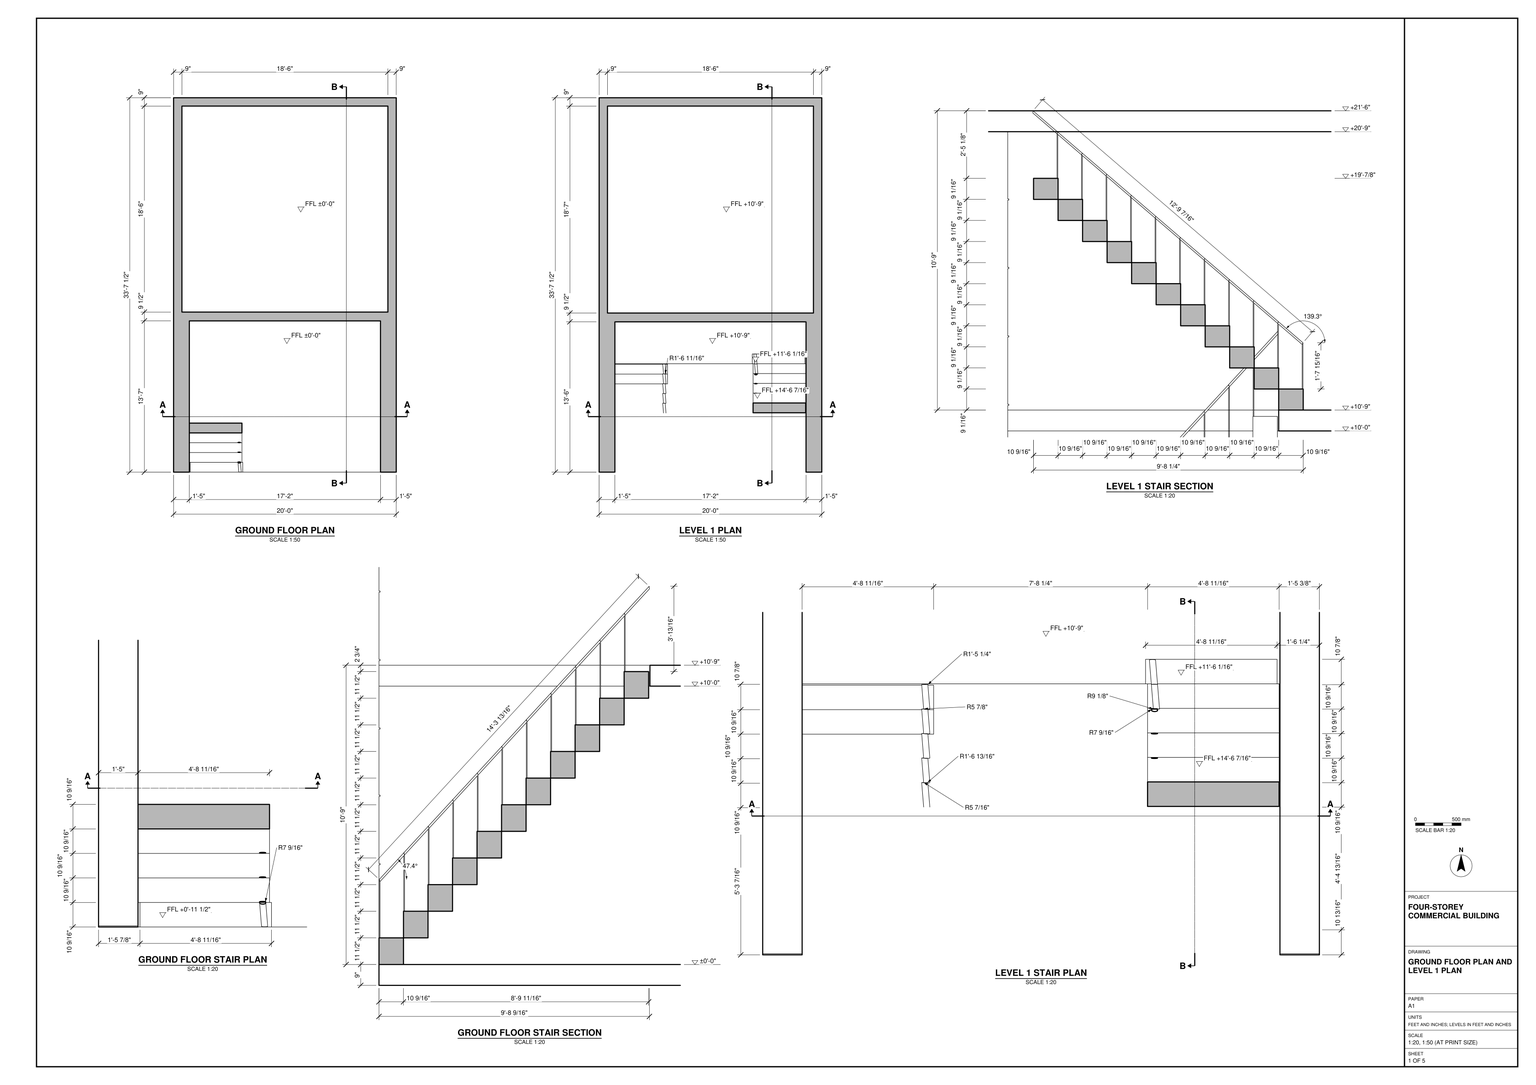
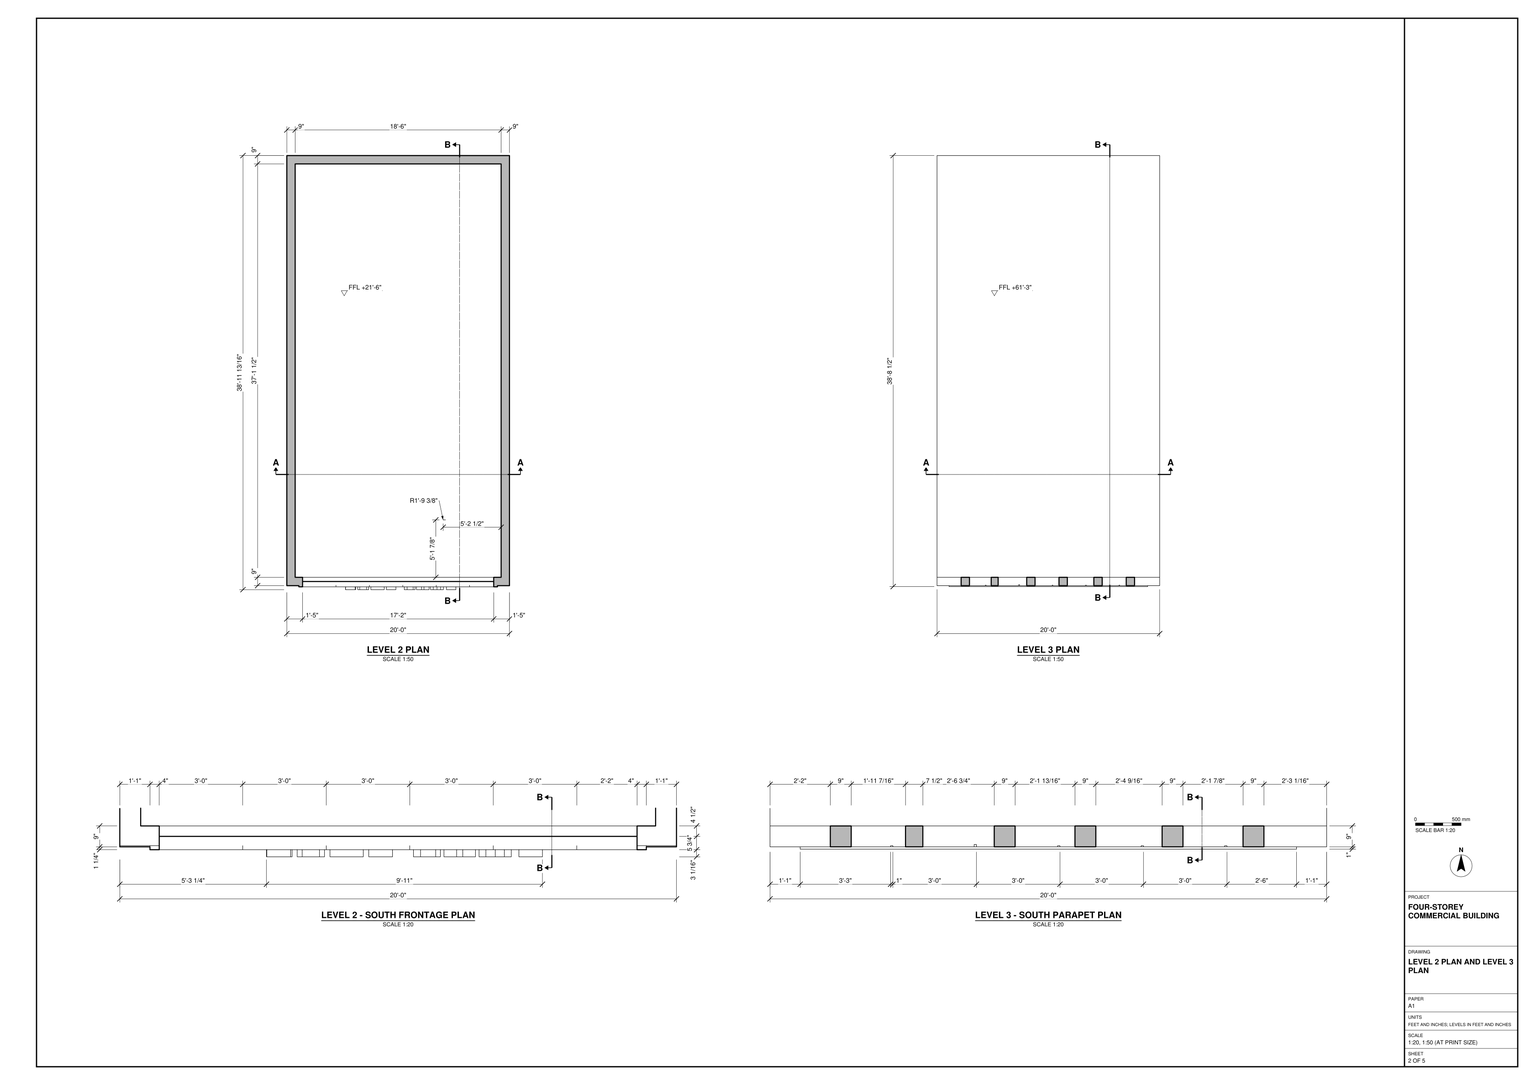
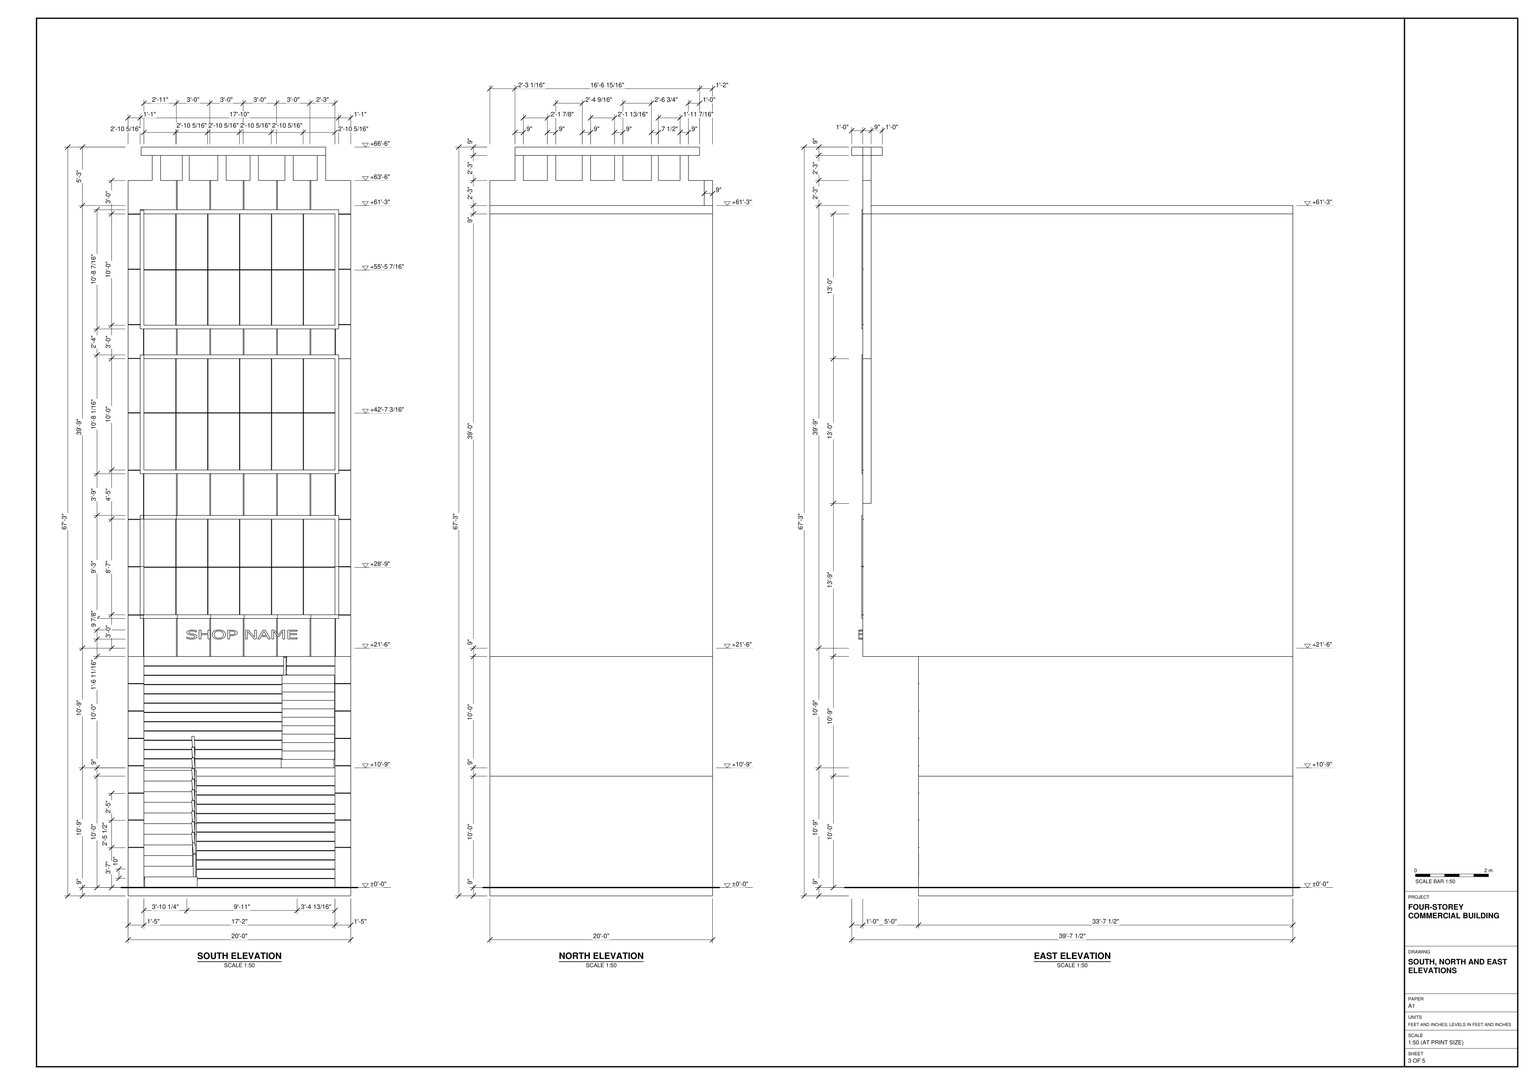
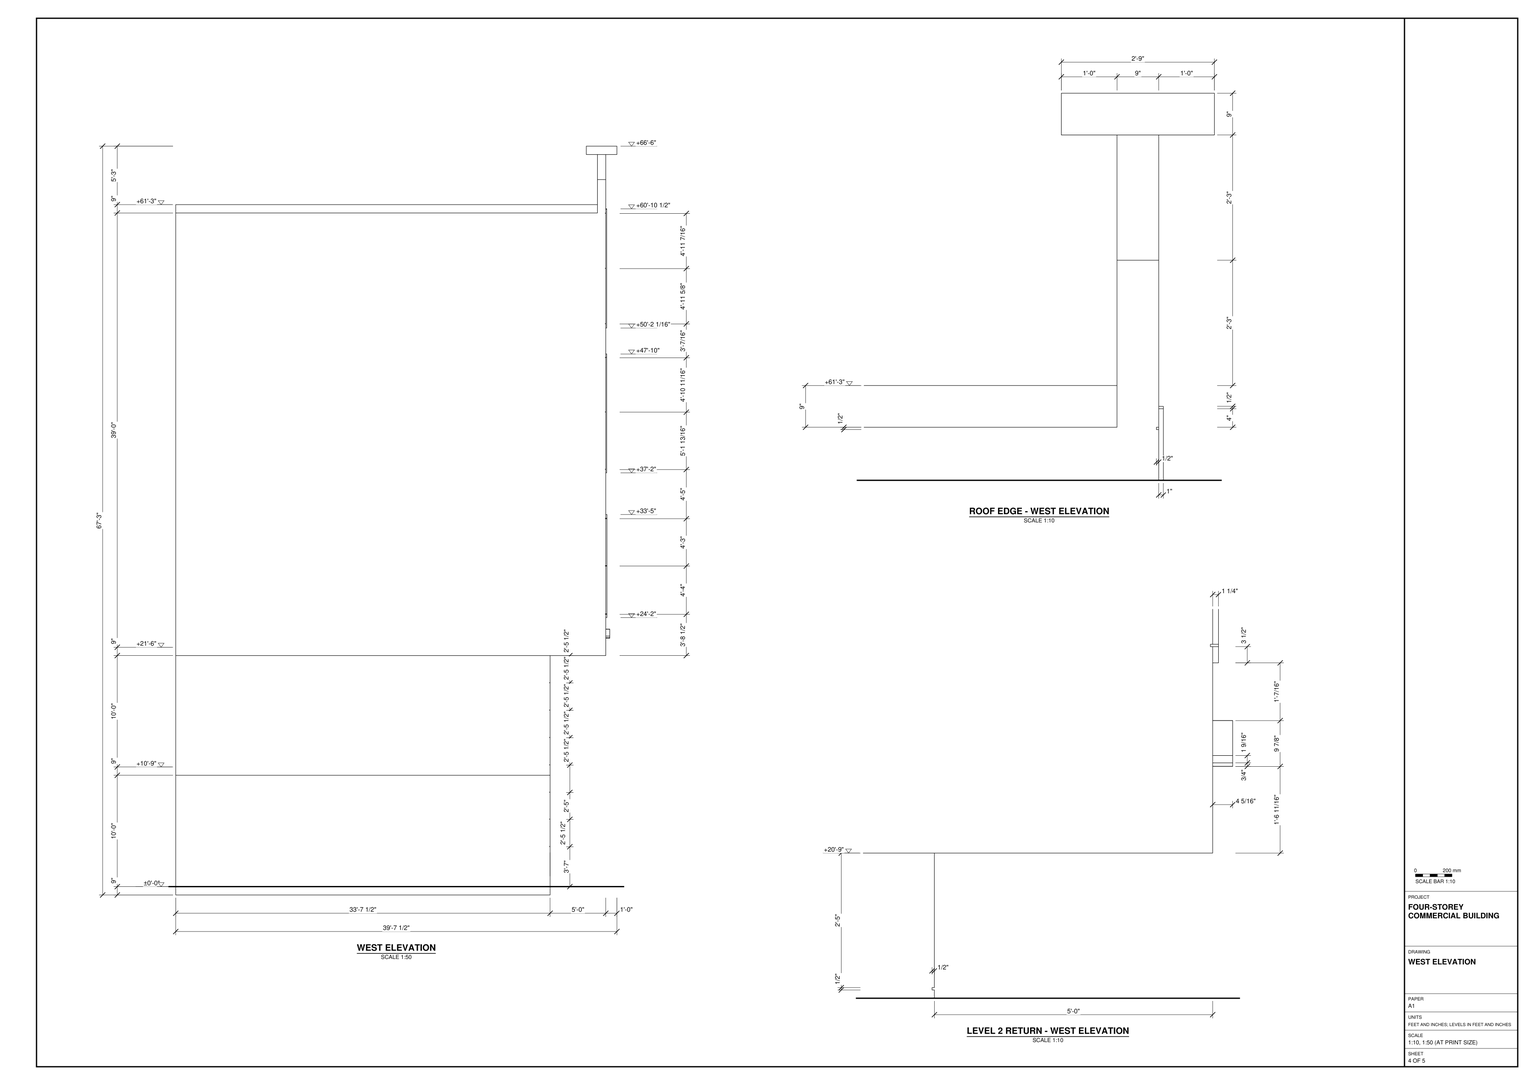
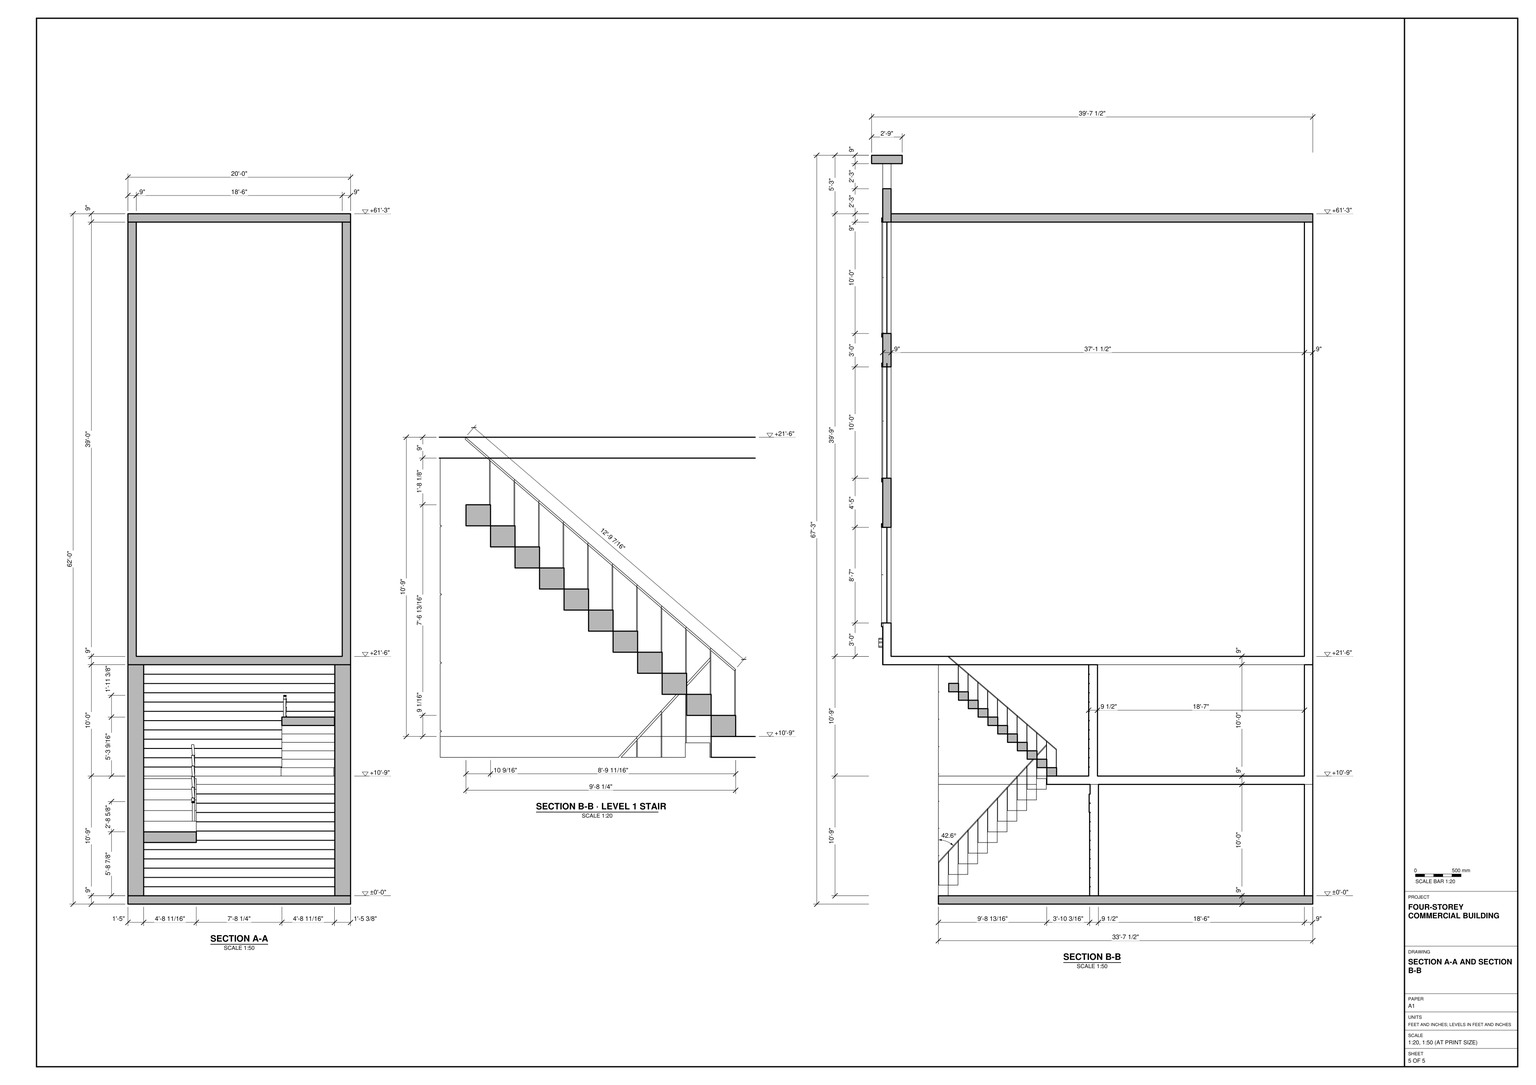
Build the commercial building in SketchUp from task_files/diagram_01.pdf. Work in feet and inches. The overall dimensions are 20'-0" across the south frontage, 39'-7 1/2" from front to back and 67'-3" from the underside of the base slab to the top of the parapet cap. Set the levels at ±0'-0", +10'-9", +21'-6" and +61'-3".

Use the ground and first-level plans to lay out the rear enclosure and the open stair bay to its south. Follow the wall thicknesses shown, including the 9" side walls around the rear space and the 1'-5" walls flanking the stair bay. Model the stair flights on the sides indicated in plan, with individual steps, landings, sloping handrails and upright supports. Use the east elevation to locate the lower setback and the upper volume that projects over it.

Model the floor slabs and flat roof. On the south face, place the shop sign in the band above the stair opening. Above it, build the three stacked glazed panels with their perimeter frames and internal divisions. Finish the south parapet with spaced uprights beneath a continuous cap. Group walls, slabs, roof and each furniture or joinery piece separately, and use components for repeated parts. Any decor or loose items shown may be suitable library components. Save one SketchUp model as output_files/four_storey_commercial_building_with_south_stair.skp.

# SketchUp Ruby script. Lengths in inches.
U = 1.inch
M = Sketchup.active_model
def pt(a) = Geom::Point3d.new(a.map { |v| v * U })
def face(e, loops, mat)
  f = e.add_face(loops[0].map { |a| pt(a) })
  loops[1..].each { |l| e.add_face(l.map { |a| pt(a) }).erase! }
  f.material = f.back_material = mat if mat
  f
end
# faces: each face lists its corners as indices into pts; further lists are holes
def faces(e, pts, list, mat = nil) = list.each { |f| face(e, (f[0].is_a?(Array) ? f : [f]).map { |l| l.map { |i| pts[i] } }, mat) }
# xy, xz, yz: faces in a plane at the given z, y or x. An outline is a flat list of corners, or four numbers for a rectangle; further outlines are holes
def ring(l) = l.size == 4 ? [[l[0], l[1]], [l[2], l[1]], [l[2], l[3]], [l[0], l[3]]] : l.each_slice(2).to_a
def flat(e, list, mat, &to3) = list.each { |f| face(e, (f[0].is_a?(Array) ? f : [f]).map { |l| ring(l).map { |u, v| to3.(u, v) } }, mat) }
def xy(e, z, list, mat = nil) = flat(e, list, mat) { |x, y| [x, y, z] }
def xz(e, y, list, mat = nil) = flat(e, list, mat) { |x, z| [x, y, z] }
def yz(e, x, list, mat = nil) = flat(e, list, mat) { |y, z| [x, y, z] }
def lines(e, pts, list) = list.each { |a, b| e.add_line(pt(pts[a]), pt(pts[b])) }
# prism: a flat outline (further loops are holes) pulled along v
def prism(e, loops, v, mat = nil)
  f = face(e, loops, mat); d = Geom::Vector3d.new(v.map { |x| x * U })
  f.pushpull(f.normal.samedirection?(d) ? d.length : -d.length)
end
def box(e, o, s, mat = nil) = prism(e, [[o, [o[0] + s[0], o[1], o[2]], [o[0] + s[0], o[1] + s[1], o[2]], [o[0], o[1] + s[1], o[2]]]], [0, 0, s[2]], mat)
def at(x, y, z, deg = 0) = Geom::Transformation.translation(pt([x, y, z])) * Geom::Transformation.rotation(ORIGIN, Z_AXIS, deg.degrees)
def axes(o, x, y, z) = Geom::Transformation.new([*x, 0, *y, 0, *z, 0, *pt(o).to_a, 1])
def part(name) = M.definitions.add(name)
# library, detail: a bought-in or finely detailed component or shape, given as its bounding box
def library(name, o, s) = part(name).tap { |d| box(d.entities, o, s) }
def detail(e, o, s) = box(e.add_group.entities, o, s)
def put(e, d, t, mat = nil) = e.add_instance(d, t).tap { |i| i.material = mat if mat }
def group(e, t, mat = nil) = e.add_group.tap { |g| g.transformation = t; g.material = mat if mat }.entities
root = M.entities
M.materials.add("Granite Dark Gray").color = [69, 68, 68]
M.materials.add("[0097_DeepSkyBlue]").color = [0, 191, 255]
M.materials.add("[0128_White]").color = [255, 255, 255]
M.materials.add("[0132_LightGray]").color = [169, 169, 169]
M.materials.add("[0134_DimGray]").color = [105, 105, 105]
M.materials.add("[0136_Charcoal]").color = [35, 35, 35]
M.materials.add("[0137_Black]").color = [0, 0, 0]
M.materials.add("[Formica Beige]").color = [211, 187, 149]
c1 = library("SHOP NAME",[0.49,0,0],[69.73,9.9,1])
c2 = part("Stair railing section")
xy(c2.entities,0,[[0,0,70.0625,99.4375]],"[0128_White]")
xy(c2.entities,31.125,[[0,0,70.0625,99.4375]],"[0132_LightGray]")
xz(c2.entities,0,[[0,0,70.0625,31.125]],"[0128_White]")
xz(c2.entities,99.4375,[[0,0,70.0625,31.125]],"[0128_White]")
yz(c2.entities,0,[[0,0,99.4375,31.125]],"[0128_White]")
yz(c2.entities,70.0625,[[0,0,99.4375,31.125]],"[0128_White]")
p = [[65.96,1.08,31.125],[66.39,1.03,31.125],[66.39,1.03,99.4],[65.96,1.08,99.35],[66.8125,1.08,31.125],[66.8125,1.08,99.36],
  [65.56,1.25,31.125],[65.56,1.25,99.23],[67.21,1.25,31.125],[67.21,1.25,99.24],[65.22,1.51,31.125],[65.22,1.51,99.03],
  [67.55,1.51,31.125],[67.55,1.51,99.05],[64.96,1.85,31.125],[64.96,1.85,98.78],[67.8125,1.85,31.125],[67.8125,1.85,98.8],
  [64.8,2.24,31.125],[64.8,2.24,98.49],[67.98,2.24,31.125],[67.98,2.24,98.51],[64.74,2.67,31.125],[64.74,2.67,98.17],
  [68.03,2.67,31.125],[68.03,2.67,98.2],[64.8,3.1,31.125],[64.8,3.1,97.86],[67.98,3.1,31.125],[67.98,3.1,97.89],
  [64.96,3.49,31.125],[64.96,3.49,97.57],[67.8125,3.49,31.125],[67.8125,3.49,97.59],[65.22,3.83,31.125],[65.22,3.83,97.32],
  [67.55,3.83,31.125],[67.55,3.83,97.34],[65.56,4.09,31.125],[65.56,4.09,97.13],[67.21,4.09,31.125],[67.21,4.09,97.15],
  [65.96,4.26,31.125],[65.96,4.26,97.02],[66.8125,4.26,31.125],[66.8125,4.26,97.02],[66.39,4.31,31.125],[66.39,4.31,96.98],
  [64.51,102.53,127.95],[64.91,102.58,127.79],[65.76,102.59,127.8],[66.16,102.54,127.96],[65.34,102.6,127.74],[64.17,102.45,128.19],
  [66.5,102.46,128.21],[63.91,102.34,128.51],[66.75,102.36,128.54],[63.74,102.22,128.89],[66.92,102.25,128.92],[63.68,102.1,129.3],
  [66.97,102.12,129.33],[63.73,101.97,129.7],[66.91,101.99,129.73],[63.89,101.85,130.08],[66.74,101.87,130.11],[64.15,101.75,130.41],
  [66.48,101.77,130.43],[64.49,101.68,130.66],[66.14,101.6875,130.68],[64.89,101.63,130.82],[65.74,101.64,130.83],[65.3125,101.62,130.88]]
faces(c2.entities,p,[[0,1,2,3],[1,4,5,2],[6,0,3,7],[4,8,9,5],[10,6,7,11],[8,12,13,9],[14,10,11,15],[12,16,17,13],
  [18,14,15,19],[16,20,21,17],[22,18,19,23],[20,24,25,21],[26,22,23,27],[24,28,29,25],[30,26,27,31],[28,32,33,29],
  [34,30,31,35],[32,36,37,33],[38,34,35,39],[36,40,41,37],[42,38,39,43],[40,44,45,41],[46,42,43,47],[44,46,47,45],
  [43,39,48,49],[41,45,50,51],[47,43,49,52],[45,47,52,50],[39,35,53,48],[37,41,51,54],[35,31,55,53],[33,37,54,56],
  [31,27,57,55],[29,33,56,58],[27,23,59,57],[25,29,58,60],[23,19,61,59],[21,25,60,62],[19,15,63,61],[17,21,62,64],
  [15,11,65,63],[13,17,64,66],[11,7,67,65],[9,13,66,68],[7,3,69,67],[5,9,68,70],[3,2,71,69],[2,5,70,71]],"[0128_White]")
c3 = part("Group\#4")
xz(c3.entities,0,[[0,0,34.33,51],[34.83,0,68.67,51],[69.17,0,103,51],[103.5,0,137.33,51],[137.83,0,171.67,51],
  [172.17,0,206,51],[0,51.5,34.33,103],[34.83,51.5,68.67,103],[69.17,51.5,103,103],[103.5,51.5,137.33,103],
  [137.83,51.5,171.67,103],[172.17,51.5,206,103]],"[0097_DeepSkyBlue]")
xz(c3.entities,0,[[34.33,0,34.83,51],[68.67,0,69.17,51],[103,0,103.5,51],[137.33,0,137.83,51],[171.67,0,172.17,51],
  [0,51,34.33,51.5],[34.33,51,34.83,51.5],[34.83,51,68.67,51.5],[68.67,51,69.17,51.5],[69.17,51,103,51.5],
  [103,51,103.5,51.5],[103.5,51,137.33,51.5],[137.33,51,137.83,51.5],[137.83,51,171.67,51.5],[171.67,51,172.17,51.5],
  [172.17,51,206,51.5],[34.33,51.5,34.83,103],[68.67,51.5,69.17,103],[103,51.5,103.5,103],[137.33,51.5,137.83,103],
  [171.67,51.5,172.17,103]],"[0137_Black]")
xy(root,-9,[[0,72,240,475.51]])
xy(root,0,[[[0,72,0,475.51,240,475.51,240,72,223,72,223,235.01,17,235.01,17,72],[9,244.51,231,466.51]],[17,72,223,235.01],[9,244.51,231,466.51]])
xy(root,9.5,[[17,235,223,235.5]])
xy(root,10,[[17,235,223,235.5]])
xy(root,19.5,[[17,235,223,235.5]])
xy(root,20,[[17,235,223,235.5]])
xy(root,29.5,[[17,235,223,235.5]])
xy(root,30,[[17,235,223,235.5]])
xy(root,39.5,[[17,235,223,235.5]])
xy(root,40,[[17,235,223,235.5]])
xy(root,43,[[0,72,17,72.5],[223,72,240,72.5]],"[Formica Beige]")
xy(root,43.5,[[0,72,17,72.5],[223,72,240,72.5]],"[Formica Beige]")
xy(root,49.5,[[17,234.99,223,235.5]])
xy(root,50,[[17,234.99,223,235.5]])
xy(root,59.5,[[17,234.99,223,235.49]])
xy(root,60,[[17,234.99,223,235.49]])
xy(root,69.5,[[17,234.99,223,235.49]])
xy(root,70,[[17,234.99,223,235.49]])
xy(root,72.5,[[0,72,17,72.5],[223,72,240,72.5]],"[Formica Beige]")
xy(root,73,[[0,72,17,72.5],[223,72,240,72.5]],"[Formica Beige]")
xy(root,79.5,[[17,234.99,223,235.49]])
xy(root,80,[[17,234.99,223,235.49]])
xy(root,89.5,[[17,234.99,223,235.49]])
xy(root,90,[[17,234.49,223,235.49]])
xy(root,99.5,[[17,234.48,223,235.48]])
xy(root,100,[[17,234.48,223,235.48]])
xy(root,101.5,[[0,72,17,72.5],[223,72,240,72.5]],"[Formica Beige]")
xy(root,102,[[0,72,17,72.5],[223,72,240,72.5]],"[Formica Beige]")
xy(root,109.5,[[17,234.48,223,235.48]])
xy(root,120,[[17,188.82,223,235.48],[9,244.51,231,466.51]])
xy(root,129,[[17,188.82,223,233.98],[9,243.48,231,466.51]])
xy(root,131,[[0,72,17,72.5],[223,72,240,72.5]],"[Formica Beige]")
xy(root,131.5,[[0,72,17,72.5],[223,72,240,72.5]],"[Formica Beige]")
xy(root,138.5,[[17,233.98,223,234.48]])
xy(root,139,[[17,233.98,223,234.48]])
xy(root,148.5,[[17,233.98,223,234.48]])
xy(root,149,[[17,233.98,223,234.48]])
xy(root,158.5,[[17,233.98,223,234.48]])
xy(root,159,[[17,233.98,223,234.48]])
xy(root,160.5,[[0,72,17,72.5],[223,72,240,72.5]],"[Formica Beige]")
xy(root,161,[[0,72,17,72.5],[223,72,240,72.5]],"[Formica Beige]")
xy(root,168.5,[[17,233.98,223,234.48]])
xy(root,169,[[17,233.98,223,234.48]])
xy(root,178.5,[[17,233.98,223,234.48]])
xy(root,179,[[17,233.98,223,234.48]])
xy(root,188.5,[[17,233.98,223,234.48]])
xy(root,189,[[17,233.98,223,234.48]])
xy(root,190,[[0,72,17,72.5],[223,72,240,72.5]],"[Formica Beige]")
xy(root,190.5,[[0,72,17,72.5],[223,72,240,72.5]],"[Formica Beige]")
xy(root,198.5,[[17,233.98,223,234.48]])
xy(root,199,[[17,233.98,223,234.48]])
xy(root,208.5,[[17,233.98,223,234.48]])
xy(root,209,[[17,233.98,223,234.48]])
xy(root,218.5,[[17,233.98,223,234.48]])
xy(root,219,[[17,233.98,223,234.48]])
xy(root,219.5,[[0,72,17,72.5]],"[0137_Black]")
xy(root,219.5,[[223,72,240,72.5]],"[Formica Beige]")
xy(root,220,[[0,72,17,72.5]],"[0137_Black]")
xy(root,220,[[223,72,240,72.5]],"[Formica Beige]")
xy(root,228.5,[[17,233.98,223,234.48]])
xy(root,229,[[17,233.98,223,234.48]])
xy(root,238.5,[[17,233.98,223,234.48]])
xy(root,239,[[17,233.98,223,234.48]])
xy(root,249,[[0,12,0,72,17,72,17,12.5,16.5,12.5,16.5,12],[17,12,17,233.98,223,233.98,223,12,197,12,197,12.5,196,12.5,196,12,161,12,161,12.5,160,12.5,160,12,125,12,125,12.5,124,12.5,124,12,89,12,89,12.5,88,12.5,88,12,53,12,53,12.5,52,12.5,52,12],[223.5,12,223.5,12.5,223,12.5,223,72,240,72,240,12],[[0,72,0,475.51,240,475.51,240,72,223,72,223,233.98,17,233.98,17,72],[9,243.48,231,466.51]]])
xy(root,258,[[9,21,231,466.51]])
xy(root,290,[[13,10.75,16.5,12],[16.5,10.75,17,12.5],[17,10.75,53,12],[53,10.75,89,12],[89,10.75,125,12],
  [125,10.75,161,12],[161,10.75,197,12],[197,10.75,227,12],[52,12,53,12.5],[88,12,89,12.5],
  [124,12,125,12.5],[160,12,161,12.5],[196,12,197,12.5],[223,12,223.5,12.5]])
xy(root,293.5,[[0,12,13,12.5],[227,12,240,12.5]])
xy(root,294,[[13,10.75,17,12.5],[17,10.75,223,21],[223,10.75,227,12.5],[0,12,13,12.5],[227,12,240,12.5]])
xy(root,345.48,[[0,12,13,12.5],[227,12,240,12.6875]])
xy(root,345.98,[[13,10.75,17,12.5],[223,10.75,227,12.6875],[0,12,13,12.5],[227,12,240,12.6875]])
xy(root,396.5,[[0,12,13,12.5],[227,12,240,12.6875]])
xy(root,397,[[13,10.75,16.5,12],[16.5,10.75,17,12],[17,10.75,52,12],[52,10.75,223,12],[0,12,13,12.5],
  [13,12,16.5,12.5],[16.5,12,17,12.5],[17,12,17,21,223,21,223,12,197,12,197,12.5,196,12.5,196,12,161,12,161,12.5,160,12.5,160,12,125,12,125,12.5,124,12.5,124,12,89,12,89,12.5,88,12.5,88,12,53,12,53,12.5,52,12.5,52,12],[223.5,12,227,12,227,12.6875,223,12.6875,223,12.5,223.5,12.5],[227,12,240,12.6875]])
xy(root,401,[[13,10.75,16.5,12],[16.5,10.75,17,12],[17,10.75,52,12],[52,10.75,227,10.75,227,12,223.5,12,223.5,12.5,223,12.5,223,12,52,12]])
xy(root,446,[[13,11,227,12]])
xy(root,449.5,[[0,12,16.5,12.5],[223.5,12,240,12.5]])
xy(root,450,[[17,11,223,12],[0,12,17,12.5],[17,12,52,12,52,12.5,53,12.5,53,12,88,12,88,12.5,89,12.5,89,12,124,12,124,12.5,125,12.5,125,12,160,12,160,12.5,161,12.5,161,12,196,12,196,12.5,197,12.5,197,12,223,12,223,21,17,21],[223,12,240,12.5]])
xy(root,511.3125,[[0,12,17,12.5]])
xy(root,511.8125,[[0,12,17,12.5]])
xy(root,570,[[17,11,223,12],[0,12,17,12.5],[17,12,17,21,223,21,223,12,197,12,197,12.5,196,12.5,196,12,161,12,161,12.5,160,12.5,160,12,125,12,125,12.5,124,12.5,124,12,89,12,89,12.5,88,12.5,88,12,53,12,53,12.5,52,12.5,52,12],[223,12,223.5,12.5],[223.5,12,223.5,12.5,223,12.5,223,21,240,21,240,12]])
xy(root,574,[[13,11,17,12]])
xy(root,574.0625,[[17,11,227,12]])
xy(root,602.0625,[[13,11,227,12]])
xy(root,606,[[17,11,223,12],[16.5,12,17,12.5],[17,12,52,12,52,12.5,53,12.5,53,12,88,12,88,12.5,89,12.5,89,12,124,12,124,12.5,125,12.5,125,12,160,12,160,12.5,161,12.5,161,12,196,12,196,12.5,197,12.5,197,12,223,12,223,21,17,21],[223,12,223.5,12.5]])
xy(root,606.4375,[[0,12,17,12.5],[223,12,240,12.5]])
xy(root,606.9375,[[0,12,17,12.5],[223,12,240,12.5]])
xy(root,666.0625,[[0,12,17,12.5],[223,12,240,12.5]])
xy(root,666.5625,[[0,12,17,12.5],[223,12,240,12.5]])
xy(root,725.5,[[0,12,17,12.5],[223,12,240,12.5]])
xy(root,726,[[17,11,223,12],[0,12,17,12.5],[17,12,17,21,223,21,223,12,197,12,197,12.5,196,12.5,196,12,161,12,161,12.5,160,12.5,160,12,125,12,125,12.5,124,12.5,124,12,89,12,89,13,88,13,88,12,53,12,53,12.5,52,12.5,52,12],[223,12,240,12.5],[223,12.5,240,21],
  [0,21,0,475.51,240,475.51,240,21,231,21,231,466.51,9,466.51,9,21],[9,21,231,466.51]])
xy(root,730,[[13,11,17,12]])
xy(root,730.5,[[13,11,227,12]])
xy(root,735,[[0,21,240,475.51]])
xy(root,762,[[0,12,26,21],[35,12,52,12,52,12.5,53,12.5,53,12,58.42,12,58.42,21,35,21],[65.89,12,88,12,88,13,89,13,89,12,96.67,12,96.67,21,65.89,21],[105.67,12,124,12,124,12.5,125,12.5,125,12,131.47,12,131.47,21,105.67,21],[140.47,12,160,12,160,12.5,161,12.5,161,12,169.04,12,169.04,21,140.47,21],
  [178.04,12,196,12,196,12.5,197,12.5,197,12,203.9375,12,203.9375,21,178.04,21],[212.9375,12,240,21]])
xy(root,789,[[14,0,26,33],[26,12,35,21],[35,12,58.42,21],[58.42,12,65.89,21],[65.89,12,212.9375,21],
  [26,21,212.9375,33]])
xy(root,789,[[26,0,212.9375,12]],"[Formica Beige]")
xy(root,798,[[14,0,212.9375,0,212.9375,12,203.9375,12,203.9375,21,212.9375,21,212.9375,33,14,33],[58.42,12,65.89,21],[96.67,12,105.67,21],[131.47,12,140.47,21],[169.04,12,178.04,21],
  [203.9375,12,212.9375,21]])
xz(root,0,[[14,789,212.9375,798]],"[Formica Beige]")
xz(root,10.75,[[13,290,16.5,293.5],[16.5,290,53,290,53,294,17,294,17,293.5,16.5,293.5],[53,290,89,294],[89,290,125,294],[125,290,161,294],
  [161,290,197,294],[197,290,227,294],[13,293.5,17,294],[13,294,17,345.98],[223,294,227,345.98],
  [13,345.98,17,397],[223,345.98,227,345.98,227,401,52,401,52,397,223,397],[13,397,16.5,401],[16.5,397,17,401],[17,397,52,401]])
xz(root,11,[[[13,446,227,446,227,574.0625,17,574.0625,17,574,13,574],[17,450,223,570]],[[13,602.0625,227,730.5],[17,606,223,726]]])
xz(root,12,[[13,397,53,401],[53,397,88,401],[88,397,89,401],[89,397,124,401],[124,397,125,401],
  [125,397,160,401],[160,397,161,401],[161,397,196,401],[196,397,197,401],[197,397,223,401],
  [223.5,397,227,401],[13,446,16.5,449.5],[16.5,446,17,446,17,450,13,450,13,449.5,16.5,449.5],[17,446,52,449.5],[52,446,53,449.5],
  [53,446,88,449.5],[88,446,89,449.5],[89,446,124,449.5],[124,446,125,449.5],[125,446,160,449.5],
  [160,446,161,449.5],[161,446,196,449.5],[196,446,197,449.5],[197,446,223,449.5],[223,446,223.5,449.5],
  [223.5,446,227,449.5],[17,449.5,52,450],[52,449.5,53,450],[53,449.5,88,450],[88,449.5,89,450],
  [89,449.5,124,450],[124,449.5,125,450],[125,449.5,160,450],[160,449.5,161,450],[161,449.5,196,450],
  [196,449.5,197,450],[197,449.5,223,450],[223,449.5,227,450],[13,450,17,511.3125],[223,450,227,569.875],
  [13,511.3125,17,511.8125],[13,511.8125,17,570],[223,569.875,227,570],[17,570,52,574.0625],[52,570,53,574.0625],
  [53,570,88,574.0625],[88,570,89,574.0625],[89,570,124,574.0625],[124,570,125,574.0625],[125,570,160,574.0625],
  [160,570,161,574.0625],[161,570,196,574.0625],[196,570,197,574.0625],[197,570,223,574.0625],[223,570,223.5,574.0625],
  [223.5,570,227,574.0625],[13,602.0625,17,606.4375],[17,602.0625,52,606],[52,602.0625,53,606],[53,602.0625,88,606],
  [88,602.0625,89,606],[89,602.0625,124,606],[124,602.0625,125,606],[125,602.0625,160,606],[160,602.0625,161,606],
  [161,602.0625,196,606],[196,602.0625,197,606],[197,602.0625,223,606],[223,602.0625,223.5,606],[223.5,602.0625,227,606.4375],
  [223,606,223.5,606.4375],[13,606.4375,17,606.9375],[223,606.4375,223.5,606.9375],[223.5,606.4375,227,606.9375],[13,606.9375,17,666.0625],
  [223,606.9375,223.5,666.0625],[223.5,606.9375,227,666.0625],[13,666.0625,17,666.5625],[223,666.0625,223.5,666.5625],[223.5,666.0625,227,666.5625],
  [13,666.5625,17,725.5],[223,666.5625,223.5,725.5],[223.5,666.5625,227,725.5],[13,725.5,17,726],[223,725.5,223.5,726],
  [223.5,725.5,227,726],[13,726,17,730],[17,726,52,726,52,730.5,13,730.5,13,730,17,730],[52,726,53,730.5],[53,726,88,730.5],
  [88,726,89,730.5],[89,726,124,730.5],[124,726,125,730.5],[125,726,160,730.5],[160,726,161,730.5],
  [161,726,196,730.5],[196,726,197,730.5],[197,726,223.5,730.5],[223.5,726,227,730.5]])
xz(root,12,[[16.5,401,17,446],[52,401,53,446],[88,401,89,446],[124,401,125,446],[160,401,161,446],
  [196,401,197,446],[227,569.875,240,570]],"[0137_Black]")
xz(root,12,[[0,249,16.5,249,16.5,290,13,290,13,293.5,0,293.5],[17,249,52,290],[53,249,88,290],[89,249,124,290],[125,249,160,290],
  [161,249,196,290],[197,249,223,290],[223.5,249,240,249,240,293.5,227,293.5,227,290,223.5,290],[0,294,13,345.48],[227,294,240,345.48],
  [0,345.98,13,396.5],[227,345.98,240,396.5],[0,397,13,397,13,401,16.5,401,16.5,446,13,446,13,449.5,0,449.5],[227,397,240,397,240,449.5,227,449.5,227,446,223.5,446,223.5,401,227,401],[17,401,52,446],
  [53,401,88,446],[89,401,124,446],[125,401,160,446],[161,401,196,446],[197,401,223,446],
  [0,450,13,511.3125],[227,450,240,569.875],[0,511.8125,13,570],[227,570,240,570,240,606.4375,227,606.4375,227,602.0625,223.5,602.0625,223.5,574.0625,227,574.0625],[0,570.375,13,570.375,13,574,17,574,17,602.0625,13,602.0625,13,606.4375,0,606.4375],
  [17,574.0625,52,602.0625],[53,574.0625,88,602.0625],[89,574.0625,124,602.0625],[125,574.0625,160,602.0625],[161,574.0625,196,602.0625],
  [197,574.0625,223,602.0625],[0,606.9375,13,666.0625],[227,606.9375,240,666.0625],[0,666.5625,13,725.5],[227,666.5625,240,725.5],
  [0,726,13,726,13,730.5,52,730.5,52,762,35,762,35,789,26,789,26,762,0,762],[227,726,240,726,240,762,212.9375,762,212.9375,789,203.9375,789,203.9375,762,197,762,197,730.5,227,730.5],[53,730.5,88,730.5,88,762,65.89,762,65.89,789,58.42,789,58.42,762,53,762],[89,730.5,124,730.5,124,762,105.67,762,105.67,789,96.67,789,96.67,762,89,762],[125,730.5,160,730.5,160,762,140.47,762,140.47,789,131.47,789,131.47,762,125,762],
  [161,730.5,196,730.5,196,762,178.04,762,178.04,789,169.04,789,169.04,762,161,762],[58.42,789,65.89,798],[96.67,789,105.67,798],[131.47,789,140.47,798],[169.04,789,178.04,798],
  [203.9375,789,212.9375,798]],"[Formica Beige]")
xz(root,12.5,[[0,345.48,13,345.98],[16.5,397,17,449.5],[52,397,53,450],[88,397,89,450],[124,397,125,450],
  [160,397,161,450],[196,397,197,450],[223,397,223.5,401],[223,449.5,240,450],[16.5,570.375,17,606],
  [223,606.4375,240,606.9375],[0,666.0625,17,666.5625],[223,666.0625,240,666.5625]])
xz(root,12.5,[[16.5,249,17,290],[52,249,53,290],[88,249,89,290],[124,249,125,290],[160,249,161,290],
  [196,249,197,290],[223,249,223.5,290],[0,293.5,13,294],[227,293.5,240,294],[0,396.5,13,397],
  [223,401,223.5,449.5],[0,449.5,17,450],[0,511.3125,17,511.8125],[0,570,17,570.375],[52,570,53,606],
  [88,570,89,606],[124,570,125,606],[160,570,161,606],[196,570,197,606],[223,570,223.5,606],
  [0,606.4375,17,606.9375],[0,725.5,17,726],[223,725.5,240,726],[52,726,53,762],[124,726,125,762],
  [160,726,161,762],[196,726,197,762]],"[0137_Black]")
xz(root,12.6875,[[223,345.98,227,346.48]])
xz(root,12.6875,[[227,345.48,240,345.98],[227,396.5,240,397]],"[0137_Black]")
xz(root,13,[[88,726,89,762]],"[0137_Black]")
xz(root,21,[[231,570,240,726],[0,726,9,735],[9,726,240,735],[0,735,9,762],[9,735,9,762,26,762,26,789,35,789,35,762,58.42,762,58.42,789,65.89,789,65.89,762,96.67,762,96.67,789,105.67,789,105.67,762,131.47,762,131.47,789,140.47,789,140.47,762,169.04,762,169.04,789,178.04,789,178.04,762,203.9375,762,203.9375,789,212.9375,789,212.9375,762,240,762,240,735],
  [58.42,789,65.89,798],[96.67,789,105.67,798],[131.47,789,140.47,798],[169.04,789,178.04,798],[203.9375,789,212.9375,798]])
xz(root,21,[[[9,258,9,726,17,726,17,606,223,606,223,726,231,726,231,258],[17,450,223,570],[17,294,223,397]]],"[0137_Black]")
xz(root,33,[[14,789,212.9375,798]])
xz(root,72,[[0,-9,240,0]])
xz(root,72,[[0,0,17,43],[223,0,240,43],[0,43.5,17,72.5],[223,43.5,240,72.5],[0,73,17,101.5],
  [223,73,240,101.5],[0,102,17,131],[223,102,240,131],[0,131.5,17,160.5],[223,131.5,240,160.5],
  [0,161,17,190],[223,161,240,190],[0,190.5,17,219.5],[223,190.5,240,219.5],[0,220,17,249],
  [223,220,240,249]],"[Formica Beige]")
xz(root,72.5,[[0,43,17,43.5],[223,43,240,43.5],[0,72.5,17,73],[223,72.5,240,73],[0,101.5,17,102],
  [223,101.5,240,102],[0,131,17,131.5],[223,131,240,131.5],[0,160.5,17,161],[223,160.5,240,161],
  [0,190,17,190.5],[223,190,240,190.5],[0,219.5,17,220],[223,219.5,240,220]],"[0137_Black]")
xz(root,188.82,[[17,120,223,129]])
xz(root,233.98,[[17,129,223,138.5],[17,139,223,148.5],[17,149,223,158.5],[17,159,223,168.5],[17,169,223,178.5],
  [17,179,223,188.5],[17,189,223,198.5],[17,199,223,208.5],[17,209,223,218.5],[17,219,223,228.5],
  [17,229,223,238.5],[17,239,223,249]],"[0134_DimGray]")
xz(root,234.48,[[17,100,223,109.5]],"[0134_DimGray]")
xz(root,234.48,[[17,138.5,223,139],[17,148.5,223,149],[17,158.5,223,159],[17,168.5,223,169],[17,178.5,223,179],
  [17,188.5,223,189],[17,198.5,223,199],[17,208.5,223,209],[17,218.5,223,219],[17,228.5,223,229],
  [17,238.5,223,239]],"[0136_Charcoal]")
xz(root,234.99,[[17,50,223,59.5],[17,60,223,69.5],[17,70,223,79.5],[17,80,223,89.5]],"[0134_DimGray]")
xz(root,235,[[17,10,223,19.5],[17,20,223,29.5],[17,30,223,39.5]],"[0134_DimGray]")
xz(root,235.48,[[17,110,223,120]],"[0134_DimGray]")
xz(root,235.48,[[17,99.5,223,100],[17,109.5,223,110]],"[0136_Charcoal]")
xz(root,235.49,[[17,59.5,223,60],[17,69.5,223,70],[17,79.5,223,80],[17,89.5,223,90]],"[0136_Charcoal]")
xz(root,235.5,[[17,9.5,223,10],[17,19.5,223,20],[17,29.5,223,30],[17,39.5,223,40],[17,49.5,223,50]],"[0136_Charcoal]")
xz(root,243.48,[[9,129,17,249],[17,129,223,249],[223,129,231,249]])
xz(root,244.51,[[9,0,231,120]])
xz(root,466.51,[[9,0,231,120],[9,129,231,249],[9,258,231,726]])
xz(root,475.51,[[0,-9,240,0],[0,0,240,120],[0,120,240,249],[0,249,240,726],[0,726,240,735]])
yz(root,0,[[72,-9,475.51,0],[72,0,72,43,72.5,43,72.5,43.5,72,43.5,72,72.5,72.5,72.5,72.5,73,72,73,72,101.5,72.5,101.5,72.5,102,72,102,72,120,475.51,120,475.51,0],[72,120,72,131,72.5,131,72.5,131.5,72,131.5,72,160.5,72.5,160.5,72.5,161,72,161,72,190,72.5,190,72.5,190.5,72,190.5,72,219.5,72.5,219.5,72.5,220,72,220,72,249,475.51,249,475.51,120],[21,726,475.51,735]])
yz(root,0,[[12,249,12,293.5,12.5,293.5,12.5,294,12,294,12,345.48,12.5,345.48,12.5,345.98,12,345.98,12,396.5,12.5,396.5,12.5,397,12,397,12,449.5,12.5,449.5,12.5,450,12,450,12,511.3125,12.5,511.3125,12.5,511.8125,12,511.8125,12,570,12.5,570,12.5,570.375,12,570.375,12,606.4375,12.5,606.4375,12.5,606.9375,12,606.9375,12,666.0625,12.5,666.0625,12.5,666.5625,12,666.5625,12,725.5,12.5,725.5,12.5,726,12,726,12,762,21,762,21,726,475.51,726,475.51,249]],"[0137_Black]")
yz(root,9,[[244.51,0,466.51,120],[243.48,129,466.51,249]])
yz(root,9,[[21,258,466.51,726]],"[0137_Black]")
yz(root,13,[[10.75,290,12,293.5],[10.75,293.5,12.5,294],[10.75,294,12,345.48],[10.75,345.48,12.5,345.98],[10.75,345.98,12,396.5],
  [10.75,396.5,12.5,397],[11,446,12,570.375],[11,570.375,12,574],[11,602.0625,12,730],[11,730,12,730.5]])
yz(root,14,[[0,789,33,798]])
yz(root,16.5,[[12,249,12.5,290],[10.75,397,12.5,397,12.5,449.5,12,449.5,12,401,10.75,401]])
yz(root,17,[[72,0,235.01,0,235,9.5,235.5,9.5,235.5,10,235,10,235,19.5,235.5,19.5,235.5,20,235,20,235,29.5,235.5,29.5,235.5,30,235,30,235,39.5,235.5,39.5,235.5,40,235,40,234.99,49.5,235.5,49.5,235.5,50,234.99,50,234.99,59.5,235.49,59.5,235.49,60,234.99,60,234.99,69.5,235.49,69.5,235.49,70,234.99,70,234.99,79.5,235.49,79.5,235.49,80,234.99,80,234.99,89.5,235.49,89.5,235.49,90,234.49,90,234.48,99.5,235.48,99.5,235.48,100,234.48,100,234.48,109.5,235.48,109.5,235.48,120,72,120,72,102,72.5,102,72.5,101.5,72,101.5,72,73,72.5,73,72.5,72.5,72,72.5,72,43.5,72.5,43.5,72.5,43,72,43],[72,120,188.82,129],[72,129,233.98,129,233.98,138.5,234.48,138.5,234.48,139,233.98,139,233.98,148.5,234.48,148.5,234.48,149,233.98,149,233.98,158.5,234.48,158.5,234.48,159,233.98,159,233.98,168.5,234.48,168.5,234.48,169,233.98,169,233.98,178.5,234.48,178.5,234.48,179,233.98,179,233.98,188.5,234.48,188.5,234.48,189,233.98,189,233.98,198.5,234.48,198.5,234.48,199,233.98,199,233.98,208.5,234.48,208.5,234.48,209,233.98,209,233.98,218.5,234.48,218.5,234.48,219,233.98,219,233.98,228.5,234.48,228.5,234.48,229,233.98,229,233.98,238.5,234.48,238.5,234.48,239,233.98,239,233.98,249,72,249,72,220,72.5,220,72.5,219.5,72,219.5,72,190.5,72.5,190.5,72.5,190,72,190,72,161,72.5,161,72.5,160.5,72,160.5,72,131.5,72.5,131.5,72.5,131,72,131],[12,249,12.5,290],[10.75,293.5,12.5,294],
  [10.75,294,21,397],[10.75,397,10.75,401,12,401,12,449.5,12.5,449.5,12.5,397],[12,449.5,12.5,450],[11,450,12,570],[12,450,21,450,21,570,12,570,12,511.8125,12.5,511.8125,12.5,511.3125,12,511.3125],
  [11,570,12,570.375],[12,570,12.5,570.375],[11,570.375,12,574],[12,570.375,12.5,606],[11,574,12,574.0625],
  [11,606,12,726],[12,606,21,606,21,726,12.5,726,12.5,725.5,12,725.5,12,666.5625,12.5,666.5625,12.5,666.0625,12,666.0625,12,606.9375,12.5,606.9375,12.5,606.4375,12,606.4375],[11,726,12,730]])
yz(root,26,[[12,762,21,789]])
yz(root,35,[[12,762,21,789]])
yz(root,52,[[12,249,12.5,290],[10.75,397,12.5,397,12.5,450,12,450,12,401,10.75,401],[12,570,12.5,606],[12,726,12.5,762]])
yz(root,53,[[12,249,12.5,290],[10.75,290,12.5,294],[12,397,12.5,450],[12,570,12.5,606],[12,726,12.5,762]])
yz(root,58.42,[[12,762,21,789],[12,789,21,798]])
yz(root,65.89,[[12,762,21,789],[12,789,21,798]])
yz(root,88,[[12,249,12.5,290],[12,397,12.5,450],[12,570,12.5,606],[12,726,13,762]])
yz(root,89,[[12,249,12.5,290],[10.75,290,12.5,294],[12,397,12.5,450],[12,570,12.5,606],[12,726,13,762]])
yz(root,96.67,[[12,762,21,798]])
yz(root,105.67,[[12,762,21,798]])
yz(root,124,[[12,249,12.5,290],[12,397,12.5,450],[12,570,12.5,606],[12,726,12.5,762]])
yz(root,125,[[12,249,12.5,290],[10.75,290,12.5,294],[12,397,12.5,450],[12,570,12.5,606],[12,726,12.5,762]])
yz(root,131.47,[[12,762,21,798]])
yz(root,140.47,[[12,762,21,798]])
yz(root,160,[[12,249,12.5,290],[12,397,12.5,450],[12,570,12.5,606],[12,726,12.5,762]])
yz(root,161,[[12,249,12.5,290],[10.75,290,12.5,294],[12,397,12.5,450],[12,570,12.5,606],[12,726,12.5,762]])
yz(root,169.04,[[12,762,21,798]])
yz(root,178.04,[[12,762,21,798]])
yz(root,196,[[12,249,12.5,290],[12,397,12.5,450],[12,570,12.5,606],[12,726,12.5,762]])
yz(root,197,[[12,249,12.5,290],[10.75,290,12.5,294],[12,397,12.5,450],[12,570,12.5,606],[12,726,12.5,762]])
yz(root,203.9375,[[12,762,21,798]])
yz(root,212.9375,[[12,762,21,789],[0,789,12,798],[12,789,21,798],[21,789,33,798]])
yz(root,223,[[72,0,72,43,72.5,43,72.5,43.5,72,43.5,72,72.5,72.5,72.5,72.5,73,72,73,72,101.5,72.5,101.5,72.5,102,72,102,72,120,235.48,120,235.48,109.5,234.48,109.5,234.48,100,235.48,100,235.48,99.5,234.48,99.5,234.49,90,235.49,90,235.49,89.5,234.99,89.5,234.99,80,235.49,80,235.49,79.5,234.99,79.5,234.99,70,235.49,70,235.49,69.5,234.99,69.5,234.99,60,235.49,60,235.49,59.5,234.99,59.5,234.99,50,235.5,50,235.5,49.5,234.99,49.5,235,40,235.5,40,235.5,39.5,235,39.5,235,30,235.5,30,235.5,29.5,235,29.5,235,20,235.5,20,235.5,19.5,235,19.5,235,10,235.5,10,235.5,9.5,235,9.5,235.01,0],[72,120,188.82,129],[72,129,72,131,72.5,131,72.5,131.5,72,131.5,72,160.5,72.5,160.5,72.5,161,72,161,72,190,72.5,190,72.5,190.5,72,190.5,72,219.5,72.5,219.5,72.5,220,72,220,72,249,233.98,249,233.98,239,234.48,239,234.48,238.5,233.98,238.5,233.98,229,234.48,229,234.48,228.5,233.98,228.5,233.98,219,234.48,219,234.48,218.5,233.98,218.5,233.98,209,234.48,209,234.48,208.5,233.98,208.5,233.98,199,234.48,199,234.48,198.5,233.98,198.5,233.98,189,234.48,189,234.48,188.5,233.98,188.5,233.98,179,234.48,179,234.48,178.5,233.98,178.5,233.98,169,234.48,169,234.48,168.5,233.98,168.5,233.98,159,234.48,159,234.48,158.5,233.98,158.5,233.98,149,234.48,149,234.48,148.5,233.98,148.5,233.98,139,234.48,139,234.48,138.5,233.98,138.5,233.98,129],[12,249,12.5,290],[10.75,294,10.75,345.98,12.6875,345.98,12.6875,346.48,10.75,346.48,10.75,397,21,397,21,294],
  [10.75,345.98,12.6875,346.48],[12,397,12.5,401],[12,401,12.5,449.5],[12,449.5,12.5,450],[11,450,12,570],
  [12,450,21,570],[12,570,12.5,606],[11,606,12,726],[12,606,12,606.4375,12.5,606.4375,12.5,606.9375,12,606.9375,12,666.0625,12.5,666.0625,12.5,666.5625,12,666.5625,12,725.5,12.5,725.5,12.5,726,21,726,21,606]])
yz(root,223.5,[[12,249,12.5,290],[12,397,12.5,401],[12,401,12.5,449.5],[12,570,12.5,606]])
yz(root,227,[[10.75,290,12,294],[12,293.5,12.5,294],[10.75,294,12,345.98],[12,345.48,12.6875,345.98],[10.75,345.98,12,346.48],
  [12,345.98,12.6875,346.48],[10.75,346.48,12,401],[12,396.5,12.6875,397],[11,446,12,574.0625],[11,602.0625,12,730.5]])
yz(root,231,[[244.51,0,466.51,120],[243.48,129,466.51,249],[21,258,466.51,726]])
yz(root,240,[[72,-9,475.51,0],[72,0,475.51,0,475.51,120,72,120,72,102,72.5,102,72.5,101.5,72,101.5,72,73,72.5,73,72.5,72.5,72,72.5,72,43.5,72.5,43.5,72.5,43,72,43],[72,120,475.51,120,475.51,249,72,249,72,220,72.5,220,72.5,219.5,72,219.5,72,190.5,72.5,190.5,72.5,190,72,190,72,161,72.5,161,72.5,160.5,72,160.5,72,131.5,72.5,131.5,72.5,131,72,131],[12,249,475.51,249,475.51,726,21,726,21,414,12,414,12,397,12.6875,397,12.6875,396.5,12,396.5,12,345.98,12.6875,345.98,12.6875,345.48,12,345.48,12,294,12.5,294,12.5,293.5,12,293.5],[12,414,21,414,21,570,12,570,12,450,12.5,450,12.5,449.5,12,449.5],
  [12,570,21,570,21,726,12.5,726,12.5,725.5,12,725.5,12,666.5625,12.5,666.5625,12.5,666.0625,12,666.0625,12,606.9375,12.5,606.9375,12.5,606.4375,12,606.4375],[12,726,21,762],[21,726,475.51,735]])
p = [[223,235.01,0],[223,235,9.5],[17,235,9.5],[17,235.01,0],[223,235,40],[223,234.99,49.5],
  [17,234.99,49.5],[17,235,40],[223,234.49,90],[223,234.48,99.5],[17,234.48,99.5],[17,234.49,90],
  [223.5,12,293.5],[223.5,12,290],[223.5,12.5,293.5],[223.5,12.5,290],[16.5,12,570.375],[16.5,12.5,570.375],
  [17,12.5,290],[17,12.5,293.5]]
faces(root,p,[[0,1,2,3],[4,5,6,7],[8,9,10,11]],"[0134_DimGray]")
lines(root,p,[[12,13],[14,15],[16,17],[18,19]])
put(root,c1,axes([62.4,12,267.68],[1.7061,0,0],[0,0,1],[0,-4.31,0]))
g1 = group(root,at(17,72,0),"[0128_White]")
put(g1,c2,axes([0,52.84,57.39],[0.80928,0,0],[0,0.10629,0],[0,0,0.36879]),"Granite Dark Gray")
put(g1,c2,axes([0,63.41,68.87],[0.80928,0,0],[0,0.10629,0],[0,0,0.36879]),"Granite Dark Gray")
put(g1,c2,axes([0,10.57,11.48],[0.80928,0,0],[0,0.10629,0],[0,0,0.36879]),"Granite Dark Gray")
put(g1,c2,axes([0,73.98,80.35],[0.80928,0,0],[0,0.10629,0],[0,0,0.36879]),"Granite Dark Gray")
put(g1,c2,axes([0,84.55,91.83],[0.80928,0,0],[0,0.10629,0],[0,0,0.36879]),"Granite Dark Gray")
put(g1,c2,axes([0,95.12,103.31],[0.80928,0,0],[0,0.10629,0],[0,0,0.36879]),"Granite Dark Gray")
put(g1,c2,axes([0,105.6875,114.79],[0.80928,0,0],[0,0.10629,0],[0,0,0.36879]),"Granite Dark Gray")
put(g1,c2,axes([0.86,0,0],[0.80928,0,0],[0,0.10629,0],[0,0,0.36879]),"Granite Dark Gray")
put(g1,c2,axes([0,31.71,34.4375],[0.80928,0,0],[0,0.10629,0],[0,0,0.36879]),"Granite Dark Gray")
put(g1,c2,axes([0,21.14,22.96],[0.80928,0,0],[0,0.10629,0],[0,0,0.36879]),"Granite Dark Gray")
put(g1,c2,axes([0,42.28,45.91],[0.80928,0,0],[0,0.10629,0],[0,0,0.36879]),"Granite Dark Gray")
g2 = group(root,at(222.62,199.39,129),"[0128_White]")
put(g2,c2,axes([0,-52.84,45.41],[-0.80928,0,0],[0,-0.10629,0],[0,0,0.29177]),"Granite Dark Gray")
put(g2,c2,axes([0,-63.41,54.49],[-0.80928,0,0],[0,-0.10629,0],[0,0,0.29177]),"Granite Dark Gray")
put(g2,c2,axes([0,-10.57,9.08],[-0.80928,0,0],[0,-0.10629,0],[0,0,0.29177]),"Granite Dark Gray")
put(g2,c2,axes([0,-73.98,63.57],[-0.80928,0,0],[0,-0.10629,0],[0,0,0.29177]),"Granite Dark Gray")
put(g2,c2,axes([0,-84.55,72.65],[-0.80928,0,0],[0,-0.10629,0],[0,0,0.29177]),"Granite Dark Gray")
put(g2,c2,axes([0,-95.12,81.73],[-0.80928,0,0],[0,-0.10629,0],[0,0,0.29177]),"Granite Dark Gray")
put(g2,c2,axes([0,-105.6875,90.8125],[-0.80928,0,0],[0,-0.10629,0],[0,0,0.29177]),"Granite Dark Gray")
put(g2,c2,axes([-0.86,0,0],[-0.80928,0,0],[0,-0.10629,0],[0,0,0.29177]),"Granite Dark Gray")
put(g2,c2,axes([0,-31.71,27.24],[-0.80928,0,0],[0,-0.10629,0],[0,0,0.29177]),"Granite Dark Gray")
put(g2,c2,axes([0,-21.14,18.16],[-0.80928,0,0],[0,-0.10629,0],[0,0,0.29177]),"Granite Dark Gray")
put(g2,c2,axes([0,-42.28,36.33],[-0.80928,0,0],[0,-0.10629,0],[0,0,0.29177]),"Granite Dark Gray")
g3 = group(root,at(17,16.5,606))
xz(g3,0,[[0,0,34.33,59.42],[34.83,0,68.67,59.42],[69.17,0,103,59.42],[103.5,0,137.33,59.42],[137.83,0,171.67,59.42],
  [172.17,0,206,59.42],[0,60,34.33,120],[34.83,60,68.67,120],[69.17,60,103,120],[103.5,60,137.33,120],
  [137.83,60,171.67,120],[172.17,60,206,120]],"[0097_DeepSkyBlue]")
xz(g3,0,[[34.33,0,34.83,59.42],[68.67,0,69.17,59.42],[103,0,103.5,59.42],[137.33,0,137.83,59.42],[171.67,0,172.17,59.42],
  [0,59.42,34.33,60],[34.33,59.42,34.83,60],[34.83,59.42,68.67,60],[68.67,59.42,69.17,60],[69.17,59.42,103,60],
  [103,59.42,103.5,60],[103.5,59.42,137.33,60],[137.33,59.42,137.83,60],[137.83,59.42,171.67,60],[171.67,59.42,172.17,60],
  [172.17,59.42,206,60],[34.33,60,34.83,120],[68.67,60,69.17,120],[103,60,103.5,120],[137.33,60,137.83,120],
  [171.67,60,172.17,120]],"[0137_Black]")
put(root,c3,at(17,16.5,294))
put(root,c3,axes([17,16.5,450],[1,0,0],[0,1,0],[0,0,1.2]))
